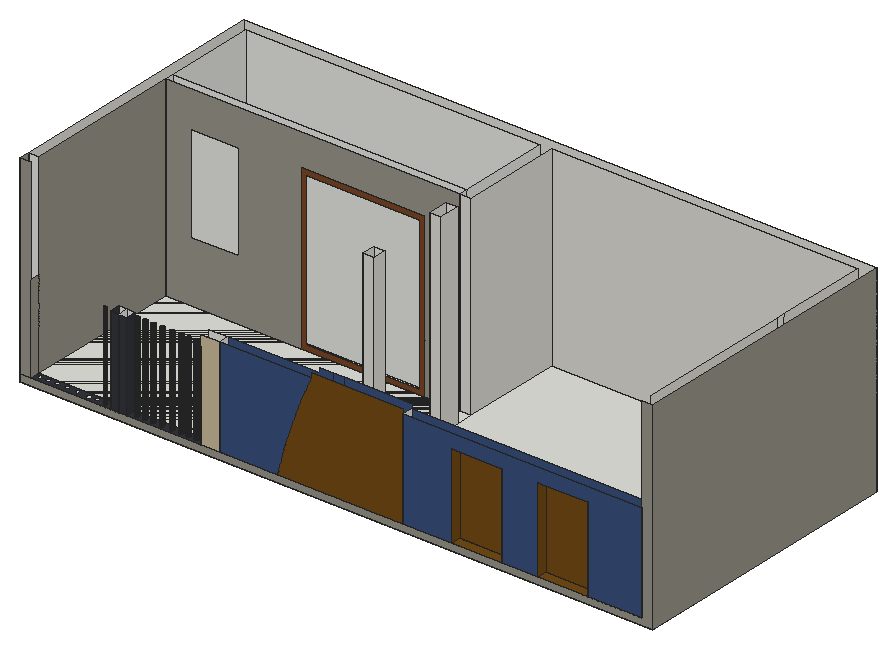
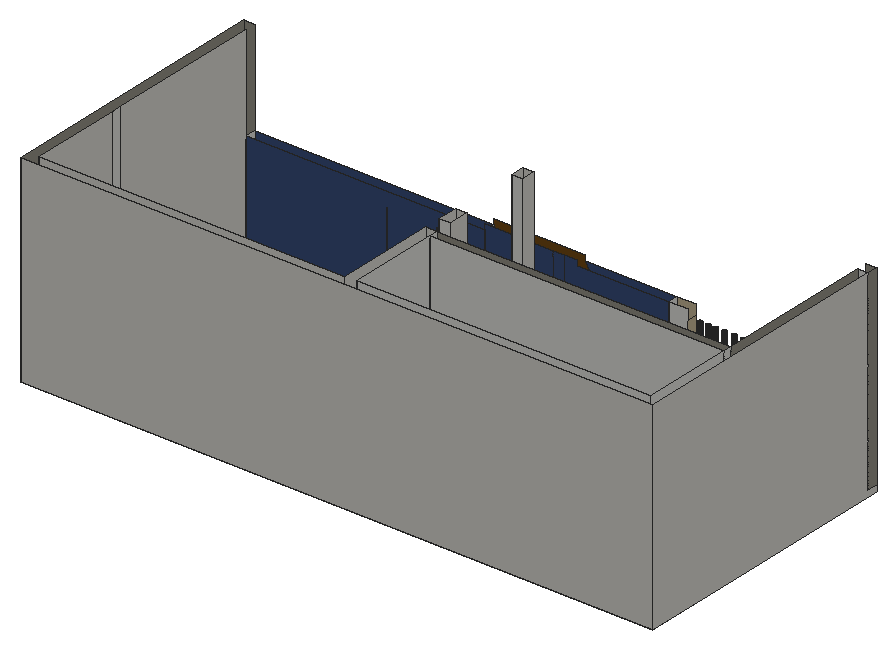
# SketchUp Ruby script. Lengths in inches.
U = 1.inch
M = Sketchup.active_model
def pt(a) = Geom::Point3d.new(a.map { |v| v * U })
def face(e, loops, mat)
  f = e.add_face(loops[0].map { |a| pt(a) })
  loops[1..].each { |l| e.add_face(l.map { |a| pt(a) }).erase! }
  f.material = f.back_material = mat if mat
  f
end
# faces: each face lists its corners as indices into pts; further lists are holes
def faces(e, pts, list, mat = nil) = list.each { |f| face(e, (f[0].is_a?(Array) ? f : [f]).map { |l| l.map { |i| pts[i] } }, mat) }
# xy, xz, yz: faces in a plane at the given z, y or x. An outline is a flat list of corners, or four numbers for a rectangle; further outlines are holes
def ring(l) = l.size == 4 ? [[l[0], l[1]], [l[2], l[1]], [l[2], l[3]], [l[0], l[3]]] : l.each_slice(2).to_a
def flat(e, list, mat, &to3) = list.each { |f| face(e, (f[0].is_a?(Array) ? f : [f]).map { |l| ring(l).map { |u, v| to3.(u, v) } }, mat) }
def xy(e, z, list, mat = nil) = flat(e, list, mat) { |x, y| [x, y, z] }
def xz(e, y, list, mat = nil) = flat(e, list, mat) { |x, z| [x, y, z] }
def yz(e, x, list, mat = nil) = flat(e, list, mat) { |y, z| [x, y, z] }
def lines(e, pts, list) = list.each { |a, b| e.add_line(pt(pts[a]), pt(pts[b])) }
# prism: a flat outline (further loops are holes) pulled along v
def prism(e, loops, v, mat = nil)
  f = face(e, loops, mat); d = Geom::Vector3d.new(v.map { |x| x * U })
  f.pushpull(f.normal.samedirection?(d) ? d.length : -d.length)
end
def box(e, o, s, mat = nil) = prism(e, [[o, [o[0] + s[0], o[1], o[2]], [o[0] + s[0], o[1] + s[1], o[2]], [o[0], o[1] + s[1], o[2]]]], [0, 0, s[2]], mat)
def at(x, y, z, deg = 0) = Geom::Transformation.translation(pt([x, y, z])) * Geom::Transformation.rotation(ORIGIN, Z_AXIS, deg.degrees)
def axes(o, x, y, z) = Geom::Transformation.new([*x, 0, *y, 0, *z, 0, *pt(o).to_a, 1])
def part(name) = M.definitions.add(name)
# library, detail: a bought-in or finely detailed component or shape, given as its bounding box
def library(name, o, s) = part(name).tap { |d| box(d.entities, o, s) }
def detail(e, o, s) = box(e.add_group.entities, o, s)
def put(e, d, t, mat = nil) = e.add_instance(d, t).tap { |i| i.material = mat if mat }
def group(e, t, mat = nil) = e.add_group.tap { |g| g.transformation = t; g.material = mat if mat }.entities
root = M.entities
M.materials.add("[Blinds Weave]").color = [114, 74, 20]
M.materials.add("[Formica Blue]").color = [58, 79, 124]
M.materials.add("[Formica Graystone]").color = [149, 146, 135]
M.materials.add("[Formica Laminate Dark]").color = [50, 53, 60]
M.materials.add("[Quartz Light Brown]").color = [199, 184, 152]
M.materials.add("[Terrazzo Tile Light]").color = [219, 217, 210]
M.materials.add("[Wood Veneer 01]").color = [120, 70, 37]
xy(root,0,[[0,18.26,843.32,391.54]])
xy(root,9,[[0,18.26,0,32.04,405.97,32.04,405.97,243,13.78,243,13.78,18.26],[120.72,18.26,131.16,32.04],[131.16,18.26,141.6,32.04],[240.76,18.26,265.93,32.04],[265.93,18.26,510.77,32.04],
  [510.77,18.26,510.77,32.04,829.54,32.04,829.54,18.26,757.4375,18.26,757.4375,31.45,690.75,31.45,690.75,18.26,642.4375,18.26,642.4375,31.76,575.75,31.76,575.75,18.26],[20.55,22.63,19.84,22.73,19.17,23,18.6,23.4375,18.17,24.01,17.89,24.67,17.8,25.38,17.89,26.09,18.17,26.76,18.6,27.33,19.17,27.76,19.84,28.04,20.55,28.13,21.26,28.04,21.92,27.76,22.49,27.33,22.93,26.76,23.2,26.09,23.3,25.38,23.2,24.67,22.93,24.01,22.49,23.4375,21.92,23,21.26,22.73],[31.74,22.63,31.02,22.73,30.36,23,29.79,23.4375,29.35,24.01,29.08,24.67,28.99,25.38,29.08,26.09,29.35,26.76,29.79,27.33,30.36,27.76,31.02,28.04,31.74,28.13,32.45,28.04,33.11,27.76,33.68,27.33,34.12,26.76,34.39,26.09,34.49,25.38,34.39,24.67,34.12,24.01,33.68,23.4375,33.11,23,32.45,22.73],[43.24,22.63,42.52,22.73,41.86,23,41.29,23.4375,40.85,24.01,40.58,24.67,40.49,25.38,40.58,26.09,40.85,26.76,41.29,27.33,41.86,27.76,42.52,28.04,43.24,28.13,43.95,28.04,44.61,27.76,45.18,27.33,45.62,26.76,45.89,26.09,45.99,25.38,45.89,24.67,45.62,24.01,45.18,23.4375,44.61,23,43.95,22.73],[56.49,22.63,55.77,22.73,55.11,23,54.54,23.4375,54.1,24.01,53.83,24.67,53.74,25.38,53.83,26.09,54.1,26.76,54.54,27.33,55.11,27.76,55.77,28.04,56.49,28.13,57.2,28.04,57.86,27.76,58.43,27.33,58.87,26.76,59.14,26.09,59.24,25.38,59.14,24.67,58.87,24.01,58.43,23.4375,57.86,23,57.2,22.73],
  [70.8,22.63,70.09,22.73,69.42,23,68.85,23.4375,68.42,24.01,68.14,24.67,68.05,25.38,68.14,26.09,68.42,26.76,68.85,27.33,69.42,27.76,70.09,28.04,70.8,28.13,71.51,28.04,72.17,27.76,72.74,27.33,73.18,26.76,73.45,26.09,73.55,25.38,73.45,24.67,73.18,24.01,72.74,23.4375,72.17,23,71.51,22.73],[86.17,22.63,85.46,22.73,84.8,23,84.23,23.4375,83.79,24.01,83.52,24.67,83.42,25.38,83.52,26.09,83.79,26.76,84.23,27.33,84.8,27.76,85.46,28.04,86.17,28.13,86.89,28.04,87.55,27.76,88.12,27.33,88.55,26.76,88.83,26.09,88.92,25.38,88.83,24.67,88.55,24.01,88.12,23.4375,87.55,23,86.89,22.73],[96.86,22.63,96.15,22.73,95.49,23,94.92,23.4375,94.48,24.01,94.2,24.67,94.11,25.38,94.2,26.09,94.48,26.76,94.92,27.33,95.49,27.76,96.15,28.04,96.86,28.13,97.57,28.04,98.24,27.76,98.81,27.33,99.24,26.76,99.52,26.09,99.61,25.38,99.52,24.67,99.24,24.01,98.81,23.4375,98.24,23,97.57,22.73],[109.61,22.63,108.9,22.73,108.24,23,107.67,23.4375,107.23,24.01,106.95,24.67,106.86,25.38,106.95,26.09,107.23,26.76,107.67,27.33,108.24,27.76,108.9,28.04,109.61,28.13,110.32,28.04,110.99,27.76,111.56,27.33,111.99,26.76,112.27,26.09,112.36,25.38,112.27,24.67,111.99,24.01,111.56,23.4375,110.99,23,110.32,22.73],[150.24,22.63,149.52,22.73,148.86,23,148.29,23.4375,147.85,24.01,147.58,24.67,147.49,25.38,147.58,26.09,147.85,26.76,148.29,27.33,148.86,27.76,149.52,28.04,150.24,28.13,150.95,28.04,151.61,27.76,152.18,27.33,152.62,26.76,152.89,26.09,152.99,25.38,152.89,24.67,152.62,24.01,152.18,23.4375,151.61,23,150.95,22.73],
  [160.92,22.63,160.21,22.73,159.55,23,158.98,23.4375,158.54,24.01,158.27,24.67,158.17,25.38,158.27,26.09,158.54,26.76,158.98,27.33,159.55,27.76,160.21,28.04,160.92,28.13,161.64,28.04,162.3,27.76,162.87,27.33,163.3,26.76,163.58,26.09,163.67,25.38,163.58,24.67,163.3,24.01,162.87,23.4375,162.3,23,161.64,22.73],[171.74,22.63,171.02,22.73,170.36,23,169.79,23.4375,169.35,24.01,169.08,24.67,168.99,25.38,169.08,26.09,169.35,26.76,169.79,27.33,170.36,27.76,171.02,28.04,171.74,28.13,172.45,28.04,173.11,27.76,173.68,27.33,174.12,26.76,174.39,26.09,174.49,25.38,174.39,24.67,174.12,24.01,173.68,23.4375,173.11,23,172.45,22.73],[183.8,22.63,183.09,22.73,182.42,23,181.85,23.4375,181.42,24.01,181.14,24.67,181.05,25.38,181.14,26.09,181.42,26.76,181.85,27.33,182.42,27.76,183.09,28.04,183.8,28.13,184.51,28.04,185.17,27.76,185.74,27.33,186.18,26.76,186.45,26.09,186.55,25.38,186.45,24.67,186.18,24.01,185.74,23.4375,185.17,23,184.51,22.73],[197.05,22.63,196.34,22.73,195.67,23,195.1,23.4375,194.67,24.01,194.39,24.67,194.3,25.38,194.39,26.09,194.67,26.76,195.1,27.33,195.67,27.76,196.34,28.04,197.05,28.13,197.76,28.04,198.42,27.76,198.99,27.33,199.43,26.76,199.7,26.09,199.8,25.38,199.7,24.67,199.43,24.01,198.99,23.4375,198.42,23,197.76,22.73],[209.17,22.63,208.46,22.73,207.8,23,207.23,23.4375,206.79,24.01,206.52,24.67,206.42,25.38,206.52,26.09,206.79,26.76,207.23,27.33,207.8,27.76,208.46,28.04,209.17,28.13,209.89,28.04,210.55,27.76,211.12,27.33,211.55,26.76,211.83,26.09,211.92,25.38,211.83,24.67,211.55,24.01,211.12,23.4375,210.55,23,209.89,22.73],
  [218.67,22.63,217.96,22.73,217.3,23,216.73,23.4375,216.29,24.01,216.02,24.67,215.92,25.38,216.02,26.09,216.29,26.76,216.73,27.33,217.3,27.76,217.96,28.04,218.67,28.13,219.39,28.04,220.05,27.76,220.62,27.33,221.05,26.76,221.33,26.09,221.42,25.38,221.33,24.67,221.05,24.01,220.62,23.4375,220.05,23,219.39,22.73],[229.92,22.63,229.21,22.73,228.55,23,227.98,23.4375,227.54,24.01,227.27,24.67,227.17,25.38,227.27,26.09,227.54,26.76,227.98,27.33,228.55,27.76,229.21,28.04,229.92,28.13,230.64,28.04,231.3,27.76,231.87,27.33,232.3,26.76,232.58,26.09,232.67,25.38,232.58,24.67,232.3,24.01,231.87,23.4375,231.3,23,230.64,22.73],[13.78,32.04,405.97,243],[405.97,32.04,421.1,82.09],[421.1,32.04,829.54,377.76],
  [405.97,82.09,421.1,100.35],[405.97,100.35,421.1,192.875],[405.97,192.875,421.1,220.7],[405.97,220.7,421.1,243],[13.78,243,405.97,255.17],
  [13.78,255.17,405.97,377.76]])
xy(root,9,[[575.75,18.26,642.4375,31.76],[690.75,18.26,757.4375,31.45]],"[Blinds Weave]")
xy(root,9,[[[13.78,18.26,120.72,32.04],[109.61,22.63,108.9,22.73,108.24,23,107.67,23.4375,107.23,24.01,106.95,24.67,106.86,25.38,106.95,26.09,107.23,26.76,107.67,27.33,108.24,27.76,108.9,28.04,109.61,28.13,110.32,28.04,110.99,27.76,111.56,27.33,111.99,26.76,112.27,26.09,112.36,25.38,112.27,24.67,111.99,24.01,111.56,23.4375,110.99,23,110.32,22.73],[20.55,22.63,19.84,22.73,19.17,23,18.6,23.4375,18.17,24.01,17.89,24.67,17.8,25.38,17.89,26.09,18.17,26.76,18.6,27.33,19.17,27.76,19.84,28.04,20.55,28.13,21.26,28.04,21.92,27.76,22.49,27.33,22.93,26.76,23.2,26.09,23.3,25.38,23.2,24.67,22.93,24.01,22.49,23.4375,21.92,23,21.26,22.73],[96.86,22.63,96.15,22.73,95.49,23,94.92,23.4375,94.48,24.01,94.2,24.67,94.11,25.38,94.2,26.09,94.48,26.76,94.92,27.33,95.49,27.76,96.15,28.04,96.86,28.13,97.57,28.04,98.24,27.76,98.81,27.33,99.24,26.76,99.52,26.09,99.61,25.38,99.52,24.67,99.24,24.01,98.81,23.4375,98.24,23,97.57,22.73],[31.74,22.63,31.02,22.73,30.36,23,29.79,23.4375,29.35,24.01,29.08,24.67,28.99,25.38,29.08,26.09,29.35,26.76,29.79,27.33,30.36,27.76,31.02,28.04,31.74,28.13,32.45,28.04,33.11,27.76,33.68,27.33,34.12,26.76,34.39,26.09,34.49,25.38,34.39,24.67,34.12,24.01,33.68,23.4375,33.11,23,32.45,22.73],[86.17,22.63,85.46,22.73,84.8,23,84.23,23.4375,83.79,24.01,83.52,24.67,83.42,25.38,83.52,26.09,83.79,26.76,84.23,27.33,84.8,27.76,85.46,28.04,86.17,28.13,86.89,28.04,87.55,27.76,88.12,27.33,88.55,26.76,88.83,26.09,88.92,25.38,88.83,24.67,88.55,24.01,88.12,23.4375,87.55,23,86.89,22.73],[43.24,22.63,42.52,22.73,41.86,23,41.29,23.4375,40.85,24.01,40.58,24.67,40.49,25.38,40.58,26.09,40.85,26.76,41.29,27.33,41.86,27.76,42.52,28.04,43.24,28.13,43.95,28.04,44.61,27.76,45.18,27.33,45.62,26.76,45.89,26.09,45.99,25.38,45.89,24.67,45.62,24.01,45.18,23.4375,44.61,23,43.95,22.73],[70.8,22.63,70.09,22.73,69.42,23,68.85,23.4375,68.42,24.01,68.14,24.67,68.05,25.38,68.14,26.09,68.42,26.76,68.85,27.33,69.42,27.76,70.09,28.04,70.8,28.13,71.51,28.04,72.17,27.76,72.74,27.33,73.18,26.76,73.45,26.09,73.55,25.38,73.45,24.67,73.18,24.01,72.74,23.4375,72.17,23,71.51,22.73],[56.49,22.63,55.77,22.73,55.11,23,54.54,23.4375,54.1,24.01,53.83,24.67,53.74,25.38,53.83,26.09,54.1,26.76,54.54,27.33,55.11,27.76,55.77,28.04,56.49,28.13,57.2,28.04,57.86,27.76,58.43,27.33,58.87,26.76,59.14,26.09,59.24,25.38,59.14,24.67,58.87,24.01,58.43,23.4375,57.86,23,57.2,22.73]],[[141.6,18.26,240.76,32.04],[229.92,22.63,229.21,22.73,228.55,23,227.98,23.4375,227.54,24.01,227.27,24.67,227.17,25.38,227.27,26.09,227.54,26.76,227.98,27.33,228.55,27.76,229.21,28.04,229.92,28.13,230.64,28.04,231.3,27.76,231.87,27.33,232.3,26.76,232.58,26.09,232.67,25.38,232.58,24.67,232.3,24.01,231.87,23.4375,231.3,23,230.64,22.73],[160.92,22.63,160.21,22.73,159.55,23,158.98,23.4375,158.54,24.01,158.27,24.67,158.17,25.38,158.27,26.09,158.54,26.76,158.98,27.33,159.55,27.76,160.21,28.04,160.92,28.13,161.64,28.04,162.3,27.76,162.87,27.33,163.3,26.76,163.58,26.09,163.67,25.38,163.58,24.67,163.3,24.01,162.87,23.4375,162.3,23,161.64,22.73],[218.67,22.63,217.96,22.73,217.3,23,216.73,23.4375,216.29,24.01,216.02,24.67,215.92,25.38,216.02,26.09,216.29,26.76,216.73,27.33,217.3,27.76,217.96,28.04,218.67,28.13,219.39,28.04,220.05,27.76,220.62,27.33,221.05,26.76,221.33,26.09,221.42,25.38,221.33,24.67,221.05,24.01,220.62,23.4375,220.05,23,219.39,22.73],[171.74,22.63,171.02,22.73,170.36,23,169.79,23.4375,169.35,24.01,169.08,24.67,168.99,25.38,169.08,26.09,169.35,26.76,169.79,27.33,170.36,27.76,171.02,28.04,171.74,28.13,172.45,28.04,173.11,27.76,173.68,27.33,174.12,26.76,174.39,26.09,174.49,25.38,174.39,24.67,174.12,24.01,173.68,23.4375,173.11,23,172.45,22.73],[209.17,22.63,208.46,22.73,207.8,23,207.23,23.4375,206.79,24.01,206.52,24.67,206.42,25.38,206.52,26.09,206.79,26.76,207.23,27.33,207.8,27.76,208.46,28.04,209.17,28.13,209.89,28.04,210.55,27.76,211.12,27.33,211.55,26.76,211.83,26.09,211.92,25.38,211.83,24.67,211.55,24.01,211.12,23.4375,210.55,23,209.89,22.73],[183.8,22.63,183.09,22.73,182.42,23,181.85,23.4375,181.42,24.01,181.14,24.67,181.05,25.38,181.14,26.09,181.42,26.76,181.85,27.33,182.42,27.76,183.09,28.04,183.8,28.13,184.51,28.04,185.17,27.76,185.74,27.33,186.18,26.76,186.45,26.09,186.55,25.38,186.45,24.67,186.18,24.01,185.74,23.4375,185.17,23,184.51,22.73],[197.05,22.63,196.34,22.73,195.67,23,195.1,23.4375,194.67,24.01,194.39,24.67,194.3,25.38,194.39,26.09,194.67,26.76,195.1,27.33,195.67,27.76,196.34,28.04,197.05,28.13,197.76,28.04,198.42,27.76,198.99,27.33,199.43,26.76,199.7,26.09,199.8,25.38,199.7,24.67,199.43,24.01,198.99,23.4375,198.42,23,197.76,22.73],[150.24,22.63,149.52,22.73,148.86,23,148.29,23.4375,147.85,24.01,147.58,24.67,147.49,25.38,147.58,26.09,147.85,26.76,148.29,27.33,148.86,27.76,149.52,28.04,150.24,28.13,150.95,28.04,151.61,27.76,152.18,27.33,152.62,26.76,152.89,26.09,152.99,25.38,152.89,24.67,152.62,24.01,152.18,23.4375,151.61,23,150.95,22.73]]],"[Formica Laminate Dark]")
xz(root,18.26,[[343.1,9,510.77,9,510.77,146.9375,388.35,146.9375,388.35,140.3125,383.67,129.71,379.15,119.04,374.8,108.29,370.6,97.49,366.58,86.62,362.72,75.69,359.03,64.71,355.5,53.66,352.14,42.57,348.96,31.43,345.94,20.24]],"[Blinds Weave]")
xz(root,18.26,[[265.93,9,343.1,9,345.94,20.24,348.96,31.43,352.14,42.57,355.5,53.66,359.03,64.71,362.72,75.69,366.58,86.62,370.6,97.49,374.8,108.29,379.15,119.04,383.67,129.71,388.35,140.3125,265.93,140.3125],[510.77,9,575.75,9,575.75,121.625,642.4375,121.625,642.4375,9,690.75,9,690.75,121.625,757.4375,121.625,757.4375,9,829.54,9,829.54,140.3125,510.77,140.3125]],"[Formica Blue]")
xz(root,18.26,[[0,0,843.32,0,843.32,267.75,829.54,267.75,829.54,9,0,9],[0,9,13.78,267.75]],"[Formica Graystone]")
xz(root,18.26,[[120.72,9,131.16,126.29],[131.16,9,141.6,126.29]],"[Formica Laminate Dark]")
xz(root,18.26,[[240.76,9,265.93,140.3125]],"[Quartz Light Brown]")
xz(root,31.45,[[690.75,9,757.4375,121.625]],"[Blinds Weave]")
xz(root,31.76,[[575.75,9,642.4375,121.625]],"[Blinds Weave]")
xz(root,32.04,[[0,9,13.78,267.75],[120.72,9,131.16,126.29],[131.16,9,141.6,126.29],[240.76,9,265.93,140.3125]])
xz(root,32.04,[[265.93,9,265.93,140.3125,388.35,140.3125,388.35,146.9375,405.97,146.9375,405.97,9],[405.97,9,421.1,146.9375],[421.1,9,510.77,146.9375],[510.77,9,829.54,140.3125]],"[Formica Blue]")
xz(root,82.09,[[405.97,9,421.1,267.75]],"[Terrazzo Tile Light]")
xz(root,100.35,[[405.97,9,421.1,267.75]])
xz(root,192.875,[[405.97,9,421.1,267.75]],"[Terrazzo Tile Light]")
xz(root,220.7,[[405.97,9,421.1,267.75]])
xz(root,243,[[[13.78,9,193.92,9,193.92,225.5,359.17,225.5,359.17,9,405.97,9,405.97,267.75,13.78,267.75],[48.09,90.32,111.9,219.95]]],"[Formica Graystone]")
xz(root,243,[[405.97,9,421.1,267.75]],"[Terrazzo Tile Light]")
xz(root,243,[[[193.92,9,359.17,225.5],[200.58,15.66,352.51,218.84]]],"[Wood Veneer 01]")
xz(root,255.17,[[13.78,9,405.97,267.75]])
xz(root,377.76,[[13.78,9,405.97,267.75]])
xz(root,377.76,[[421.1,9,829.54,267.75]],"[Terrazzo Tile Light]")
xz(root,391.54,[[0,0,843.32,267.75]],"[Terrazzo Tile Light]")
yz(root,0,[[18.26,9,32.04,267.75]],"[Formica Graystone]")
yz(root,0,[[18.26,0,18.26,9,32.04,9,32.04,267.75,391.54,267.75,391.54,0]],"[Terrazzo Tile Light]")
yz(root,13.78,[[243,9,255.17,267.75],[255.17,9,377.76,267.75]])
yz(root,13.78,[[18.26,9,32.04,126.29],[32.04,9,243,267.75]],"[Formica Graystone]")
yz(root,120.72,[[18.26,9,32.04,126.29]],"[Formica Laminate Dark]")
yz(root,131.16,[[18.26,9,32.04,126.29]])
yz(root,141.6,[[18.26,9,32.04,126.29]],"[Formica Laminate Dark]")
yz(root,240.76,[[18.26,9,32.04,126.29]],"[Quartz Light Brown]")
yz(root,265.93,[[18.26,9,32.04,140.3125]])
yz(root,405.97,[[243,9,255.17,267.75],[255.17,9,377.76,267.75]])
yz(root,405.97,[[82.09,9,100.35,267.75],[192.875,9,220.7,267.75]],"[Terrazzo Tile Light]")
yz(root,421.1,[[82.09,9,100.35,267.75],[192.875,9,220.7,267.75],[243,9,377.76,267.75]],"[Terrazzo Tile Light]")
yz(root,510.77,[[18.26,9,32.04,140.3125]])
yz(root,575.75,[[18.26,9,31.76,121.625]],"[Blinds Weave]")
yz(root,642.4375,[[18.26,9,31.76,121.625]],"[Blinds Weave]")
yz(root,690.75,[[18.26,9,31.45,121.625]],"[Blinds Weave]")
yz(root,757.4375,[[18.26,9,31.45,121.625]],"[Blinds Weave]")
yz(root,829.54,[[18.26,9,32.04,140.3125],[243,9,255.17,267.75]])
yz(root,829.54,[[32.04,9,243,267.75],[255.17,9,377.76,267.75]],"[Terrazzo Tile Light]")
yz(root,843.32,[[18.26,0,391.54,267.75]],"[Formica Graystone]")
p = [[108.9,22.73,9],[109.61,22.63,9],[109.61,22.63,126.29],[108.9,22.73,126.29],[110.32,22.73,9],[110.32,22.73,126.29],
  [149.52,22.73,9],[150.24,22.63,9],[150.24,22.63,126.29],[149.52,22.73,126.29],[150.95,22.73,9],[150.95,22.73,126.29],
  [160.21,22.73,9],[160.92,22.63,9],[160.92,22.63,126.29],[160.21,22.73,126.29],[161.64,22.73,9],[161.64,22.73,126.29],
  [171.02,22.73,9],[171.74,22.63,9],[171.74,22.63,126.29],[171.02,22.73,126.29],[172.45,22.73,9],[172.45,22.73,126.29],
  [183.09,22.73,9],[183.8,22.63,9],[183.8,22.63,126.29],[183.09,22.73,126.29],[184.51,22.73,9],[184.51,22.73,126.29],
  [196.34,22.73,9],[197.05,22.63,9],[197.05,22.63,126.29],[196.34,22.73,126.29],[197.76,22.73,9],[197.76,22.73,126.29],
  [208.46,22.73,9],[209.17,22.63,9],[209.17,22.63,126.29],[208.46,22.73,126.29],[209.89,22.73,9],[209.89,22.73,126.29],
  [217.96,22.73,9],[218.67,22.63,9],[218.67,22.63,126.29],[217.96,22.73,126.29],[219.39,22.73,9],[219.39,22.73,126.29],
  [229.21,22.73,9],[229.92,22.63,9],[229.92,22.63,126.29],[229.21,22.73,126.29],[230.64,22.73,9],[230.64,22.73,126.29],
  [108.24,23,9],[108.24,23,126.29],[110.99,23,9],[110.99,23,126.29],[148.86,23,9],[148.86,23,126.29],
  [151.61,23,9],[151.61,23,126.29],[159.55,23,9],[159.55,23,126.29],[162.3,23,9],[162.3,23,126.29],
  [170.36,23,9],[170.36,23,126.29],[173.11,23,9],[173.11,23,126.29],[182.42,23,9],[182.42,23,126.29],
  [185.17,23,9],[185.17,23,126.29],[195.67,23,9],[195.67,23,126.29],[198.42,23,9],[198.42,23,126.29],
  [207.8,23,9],[207.8,23,126.29],[210.55,23,9],[210.55,23,126.29],[217.3,23,9],[217.3,23,126.29],
  [220.05,23,9],[220.05,23,126.29],[228.55,23,9],[228.55,23,126.29],[231.3,23,9],[231.3,23,126.29],
  [111.56,23.4375,9],[111.56,23.4375,126.29],[148.29,23.4375,9],[148.29,23.4375,126.29],[152.18,23.4375,9],[152.18,23.4375,126.29],
  [158.98,23.4375,9],[158.98,23.4375,126.29],[162.87,23.4375,9],[162.87,23.4375,126.29],[169.79,23.4375,9],[169.79,23.4375,126.29],
  [173.68,23.4375,9],[173.68,23.4375,126.29],[181.85,23.4375,9],[181.85,23.4375,126.29],[185.74,23.4375,9],[185.74,23.4375,126.29],
  [195.1,23.4375,9],[195.1,23.4375,126.29],[198.99,23.4375,9],[198.99,23.4375,126.29],[207.23,23.4375,9],[207.23,23.4375,126.29],
  [211.12,23.4375,9],[211.12,23.4375,126.29],[216.73,23.4375,9],[216.73,23.4375,126.29],[220.62,23.4375,9],[220.62,23.4375,126.29],
  [227.98,23.4375,9],[227.98,23.4375,126.29],[231.87,23.4375,9],[231.87,23.4375,126.29],[147.85,24.01,9],[147.85,24.01,126.29],
  [152.62,24.01,9],[152.62,24.01,126.29],[158.54,24.01,9],[158.54,24.01,126.29],[163.3,24.01,9],[163.3,24.01,126.29],
  [169.35,24.01,9],[169.35,24.01,126.29],[174.12,24.01,9],[174.12,24.01,126.29],[181.42,24.01,9],[181.42,24.01,126.29],
  [186.18,24.01,9],[186.18,24.01,126.29],[194.67,24.01,9],[194.67,24.01,126.29],[199.43,24.01,9],[199.43,24.01,126.29],
  [206.79,24.01,9],[206.79,24.01,126.29],[211.55,24.01,9],[211.55,24.01,126.29],[216.29,24.01,9],[216.29,24.01,126.29],
  [221.05,24.01,9],[221.05,24.01,126.29],[227.54,24.01,9],[227.54,24.01,126.29],[232.3,24.01,9],[232.3,24.01,126.29],
  [147.58,24.67,9],[147.58,24.67,126.29],[152.89,24.67,9],[152.89,24.67,126.29],[158.27,24.67,9],[158.27,24.67,126.29],
  [163.58,24.67,9],[163.58,24.67,126.29],[169.08,24.67,9],[169.08,24.67,126.29],[174.39,24.67,9],[174.39,24.67,126.29],
  [181.14,24.67,9],[181.14,24.67,126.29],[186.45,24.67,9],[186.45,24.67,126.29],[194.39,24.67,9],[194.39,24.67,126.29],
  [199.7,24.67,9],[199.7,24.67,126.29],[206.52,24.67,9],[206.52,24.67,126.29],[211.83,24.67,9],[211.83,24.67,126.29],
  [216.02,24.67,9],[216.02,24.67,126.29],[221.33,24.67,9],[221.33,24.67,126.29],[227.27,24.67,9],[227.27,24.67,126.29],
  [232.58,24.67,9],[232.58,24.67,126.29],[147.49,25.38,9],[147.49,25.38,126.29],[152.99,25.38,9],[152.99,25.38,126.29],
  [158.17,25.38,9],[158.17,25.38,126.29],[163.67,25.38,9],[163.67,25.38,126.29],[168.99,25.38,9],[168.99,25.38,126.29],
  [174.49,25.38,9],[174.49,25.38,126.29],[181.05,25.38,9],[181.05,25.38,126.29],[186.55,25.38,9],[186.55,25.38,126.29],
  [194.3,25.38,9],[194.3,25.38,126.29],[199.8,25.38,9],[199.8,25.38,126.29],[206.42,25.38,9],[206.42,25.38,126.29],
  [211.92,25.38,9],[211.92,25.38,126.29],[215.92,25.38,9],[215.92,25.38,126.29],[221.42,25.38,9],[221.42,25.38,126.29],
  [227.17,25.38,9],[227.17,25.38,126.29],[232.67,25.38,9],[232.67,25.38,126.29],[147.58,26.09,9],[147.58,26.09,126.29],
  [152.89,26.09,9],[152.89,26.09,126.29],[158.27,26.09,9],[158.27,26.09,126.29],[163.58,26.09,9],[163.58,26.09,126.29],
  [169.08,26.09,9],[169.08,26.09,126.29],[174.39,26.09,9],[174.39,26.09,126.29],[181.14,26.09,9],[181.14,26.09,126.29],
  [186.45,26.09,9],[186.45,26.09,126.29],[194.39,26.09,9],[194.39,26.09,126.29],[199.7,26.09,9],[199.7,26.09,126.29],
  [206.52,26.09,9],[206.52,26.09,126.29],[211.83,26.09,9],[211.83,26.09,126.29],[216.02,26.09,9],[216.02,26.09,126.29],
  [221.33,26.09,9],[221.33,26.09,126.29],[227.27,26.09,9],[227.27,26.09,126.29],[232.58,26.09,9],[232.58,26.09,126.29],
  [147.85,26.76,9],[147.85,26.76,126.29],[152.62,26.76,9],[152.62,26.76,126.29],[158.54,26.76,9],[158.54,26.76,126.29],
  [163.3,26.76,9],[163.3,26.76,126.29],[169.35,26.76,9],[169.35,26.76,126.29],[174.12,26.76,9],[174.12,26.76,126.29],
  [181.42,26.76,9],[181.42,26.76,126.29],[186.18,26.76,9],[186.18,26.76,126.29],[194.67,26.76,9],[194.67,26.76,126.29],
  [199.43,26.76,9],[199.43,26.76,126.29],[206.79,26.76,9],[206.79,26.76,126.29],[211.55,26.76,9],[211.55,26.76,126.29],
  [216.29,26.76,9],[216.29,26.76,126.29],[221.05,26.76,9],[221.05,26.76,126.29],[227.54,26.76,9],[227.54,26.76,126.29],
  [232.3,26.76,9],[232.3,26.76,126.29],[148.29,27.33,9],[148.29,27.33,126.29],[152.18,27.33,9],[152.18,27.33,126.29],
  [158.98,27.33,9],[158.98,27.33,126.29],[162.87,27.33,9],[162.87,27.33,126.29],[169.79,27.33,9],[169.79,27.33,126.29],
  [173.68,27.33,9],[173.68,27.33,126.29],[181.85,27.33,9],[181.85,27.33,126.29],[185.74,27.33,9],[185.74,27.33,126.29],
  [195.1,27.33,9],[195.1,27.33,126.29],[198.99,27.33,9],[198.99,27.33,126.29],[207.23,27.33,9],[207.23,27.33,126.29],
  [211.12,27.33,9],[211.12,27.33,126.29],[216.73,27.33,9],[216.73,27.33,126.29],[220.62,27.33,9],[220.62,27.33,126.29],
  [227.98,27.33,9],[227.98,27.33,126.29],[231.87,27.33,9],[231.87,27.33,126.29],[148.86,27.76,9],[148.86,27.76,126.29],
  [151.61,27.76,9],[151.61,27.76,126.29],[159.55,27.76,9],[159.55,27.76,126.29],[162.3,27.76,9],[162.3,27.76,126.29],
  [170.36,27.76,9],[170.36,27.76,126.29],[173.11,27.76,9],[173.11,27.76,126.29],[182.42,27.76,9],[182.42,27.76,126.29],
  [185.17,27.76,9],[185.17,27.76,126.29],[195.67,27.76,9],[195.67,27.76,126.29],[198.42,27.76,9],[198.42,27.76,126.29],
  [207.8,27.76,9],[207.8,27.76,126.29],[210.55,27.76,9],[210.55,27.76,126.29],[217.3,27.76,9],[217.3,27.76,126.29],
  [220.05,27.76,9],[220.05,27.76,126.29],[228.55,27.76,9],[228.55,27.76,126.29],[231.3,27.76,9],[231.3,27.76,126.29],
  [149.52,28.04,9],[149.52,28.04,126.29],[150.95,28.04,9],[150.95,28.04,126.29],[160.21,28.04,9],[160.21,28.04,126.29],
  [161.64,28.04,9],[161.64,28.04,126.29],[171.02,28.04,9],[171.02,28.04,126.29],[172.45,28.04,9],[172.45,28.04,126.29],
  [183.09,28.04,9],[183.09,28.04,126.29],[184.51,28.04,9],[184.51,28.04,126.29],[196.34,28.04,9],[196.34,28.04,126.29],
  [197.76,28.04,9],[197.76,28.04,126.29],[208.46,28.04,9],[208.46,28.04,126.29],[209.89,28.04,9],[209.89,28.04,126.29],
  [217.96,28.04,9],[217.96,28.04,126.29],[219.39,28.04,9],[219.39,28.04,126.29],[229.21,28.04,9],[229.21,28.04,126.29],
  [230.64,28.04,9],[230.64,28.04,126.29],[150.24,28.13,9],[150.24,28.13,126.29],[160.92,28.13,9],[160.92,28.13,126.29],
  [171.74,28.13,9],[171.74,28.13,126.29],[183.8,28.13,9],[183.8,28.13,126.29],[197.05,28.13,9],[197.05,28.13,126.29],
  [209.17,28.13,9],[209.17,28.13,126.29],[218.67,28.13,9],[218.67,28.13,126.29],[229.92,28.13,9],[229.92,28.13,126.29]]
faces(root,p,[[0,1,2,3],[1,4,5,2],[6,7,8,9],[7,10,11,8],[12,13,14,15],[13,16,17,14],[18,19,20,21],[19,22,23,20],
  [24,25,26,27],[25,28,29,26],[30,31,32,33],[31,34,35,32],[36,37,38,39],[37,40,41,38],[42,43,44,45],[43,46,47,44],
  [48,49,50,51],[49,52,53,50],[54,0,3,55],[4,56,57,5],[58,6,9,59],[10,60,61,11],[62,12,15,63],[16,64,65,17],
  [66,18,21,67],[22,68,69,23],[70,24,27,71],[28,72,73,29],[74,30,33,75],[34,76,77,35],[78,36,39,79],[40,80,81,41],
  [82,42,45,83],[46,84,85,47],[86,48,51,87],[52,88,89,53],[56,90,91,57],[92,58,59,93],[60,94,95,61],[96,62,63,97],
  [64,98,99,65],[100,66,67,101],[68,102,103,69],[104,70,71,105],[72,106,107,73],[108,74,75,109],[76,110,111,77],[112,78,79,113],
  [80,114,115,81],[116,82,83,117],[84,118,119,85],[120,86,87,121],[88,122,123,89],[124,92,93,125],[94,126,127,95],[128,96,97,129],
  [98,130,131,99],[132,100,101,133],[102,134,135,103],[136,104,105,137],[106,138,139,107],[140,108,109,141],[110,142,143,111],[144,112,113,145],
  [114,146,147,115],[148,116,117,149],[118,150,151,119],[152,120,121,153],[122,154,155,123],[156,124,125,157],[126,158,159,127],[160,128,129,161],
  [130,162,163,131],[164,132,133,165],[134,166,167,135],[168,136,137,169],[138,170,171,139],[172,140,141,173],[142,174,175,143],[176,144,145,177],
  [146,178,179,147],[180,148,149,181],[150,182,183,151],[184,152,153,185],[154,186,187,155],[188,156,157,189],[158,190,191,159],[192,160,161,193],
  [162,194,195,163],[196,164,165,197],[166,198,199,167],[200,168,169,201],[170,202,203,171],[204,172,173,205],[174,206,207,175],[208,176,177,209],
  [178,210,211,179],[212,180,181,213],[182,214,215,183],[216,184,185,217],[186,218,219,187],[220,188,189,221],[190,222,223,191],[224,192,193,225],
  [194,226,227,195],[228,196,197,229],[198,230,231,199],[232,200,201,233],[202,234,235,203],[236,204,205,237],[206,238,239,207],[240,208,209,241],
  [210,242,243,211],[244,212,213,245],[214,246,247,215],[248,216,217,249],[218,250,251,219],[252,220,221,253],[222,254,255,223],[256,224,225,257],
  [226,258,259,227],[260,228,229,261],[230,262,263,231],[264,232,233,265],[234,266,267,235],[268,236,237,269],[238,270,271,239],[272,240,241,273],
  [242,274,275,243],[276,244,245,277],[246,278,279,247],[280,248,249,281],[250,282,283,251],[284,252,253,285],[254,286,287,255],[288,256,257,289],
  [258,290,291,259],[292,260,261,293],[262,294,295,263],[296,264,265,297],[266,298,299,267],[300,268,269,301],[270,302,303,271],[304,272,273,305],
  [274,306,307,275],[308,276,277,309],[278,310,311,279],[312,280,281,313],[282,314,315,283],[316,284,285,317],[286,318,319,287],[320,288,289,321],
  [290,322,323,291],[324,292,293,325],[294,326,327,295],[328,296,297,329],[298,330,331,299],[332,300,301,333],[302,334,335,303],[336,304,305,337],
  [306,338,339,307],[340,308,309,341],[310,342,343,311],[344,312,313,345],[314,346,347,315],[348,316,317,349],[318,350,351,319],[352,320,321,353],
  [322,354,355,323],[356,324,325,357],[326,358,359,327],[360,328,329,361],[330,362,363,331],[364,332,333,365],[334,366,367,335],[368,336,337,369],
  [338,370,371,339],[372,340,341,373],[342,374,375,343],[376,344,345,377],[346,378,379,347],[380,348,349,381],[350,380,381,351],[382,352,353,383],
  [354,382,383,355],[384,356,357,385],[358,384,385,359],[386,360,361,387],[362,386,387,363],[388,364,365,389],[366,388,389,367],[390,368,369,391],
  [370,390,391,371],[392,372,373,393],[374,392,393,375],[394,376,377,395],[378,394,395,379]],"[Formica Laminate Dark]")
